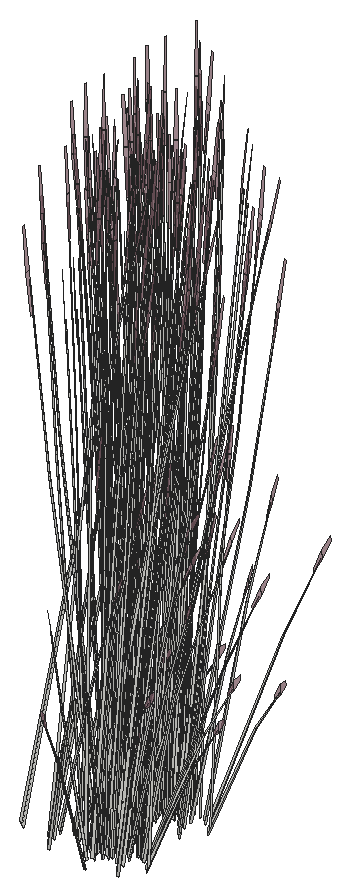
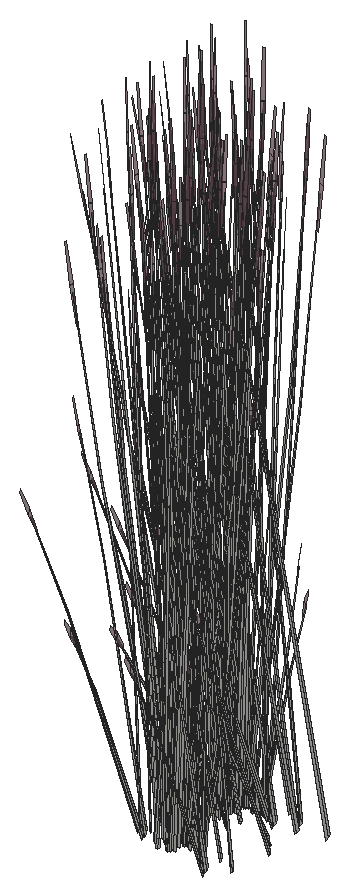
# SketchUp Ruby script. Lengths in inches.
U = 1.inch
M = Sketchup.active_model
def pt(a) = Geom::Point3d.new(a.map { |v| v * U })
def face(e, loops, mat)
  f = e.add_face(loops[0].map { |a| pt(a) })
  loops[1..].each { |l| e.add_face(l.map { |a| pt(a) }).erase! }
  f.material = f.back_material = mat if mat
  f
end
# faces: each face lists its corners as indices into pts; further lists are holes
def faces(e, pts, list, mat = nil) = list.each { |f| face(e, (f[0].is_a?(Array) ? f : [f]).map { |l| l.map { |i| pts[i] } }, mat) }
# xy, xz, yz: faces in a plane at the given z, y or x. An outline is a flat list of corners, or four numbers for a rectangle; further outlines are holes
def ring(l) = l.size == 4 ? [[l[0], l[1]], [l[2], l[1]], [l[2], l[3]], [l[0], l[3]]] : l.each_slice(2).to_a
def flat(e, list, mat, &to3) = list.each { |f| face(e, (f[0].is_a?(Array) ? f : [f]).map { |l| ring(l).map { |u, v| to3.(u, v) } }, mat) }
def xy(e, z, list, mat = nil) = flat(e, list, mat) { |x, y| [x, y, z] }
def xz(e, y, list, mat = nil) = flat(e, list, mat) { |x, z| [x, y, z] }
def yz(e, x, list, mat = nil) = flat(e, list, mat) { |y, z| [x, y, z] }
def lines(e, pts, list) = list.each { |a, b| e.add_line(pt(pts[a]), pt(pts[b])) }
# prism: a flat outline (further loops are holes) pulled along v
def prism(e, loops, v, mat = nil)
  f = face(e, loops, mat); d = Geom::Vector3d.new(v.map { |x| x * U })
  f.pushpull(f.normal.samedirection?(d) ? d.length : -d.length)
end
def box(e, o, s, mat = nil) = prism(e, [[o, [o[0] + s[0], o[1], o[2]], [o[0] + s[0], o[1] + s[1], o[2]], [o[0], o[1] + s[1], o[2]]]], [0, 0, s[2]], mat)
def at(x, y, z, deg = 0) = Geom::Transformation.translation(pt([x, y, z])) * Geom::Transformation.rotation(ORIGIN, Z_AXIS, deg.degrees)
def axes(o, x, y, z) = Geom::Transformation.new([*x, 0, *y, 0, *z, 0, *pt(o).to_a, 1])
def part(name) = M.definitions.add(name)
# library, detail: a bought-in or finely detailed component or shape, given as its bounding box
def library(name, o, s) = part(name).tap { |d| box(d.entities, o, s) }
def detail(e, o, s) = box(e.add_group.entities, o, s)
def put(e, d, t, mat = nil) = e.add_instance(d, t).tap { |i| i.material = mat if mat }
def group(e, t, mat = nil) = e.add_group.tap { |g| g.transformation = t; g.material = mat if mat }.entities
root = M.entities
M.materials.add("LightPink_Translucent").color = [144, 107, 117]
M.materials["LightPink_Translucent"].alpha = 0.75
c1 = part("blade")
p = [[2.15,0.21,22],[0,0.17,0],[0.09,0.45,0],[2.18,0.31,22],[2.29,0.31,22],[0.38,0.45,0],
  [2.48,0.24,33],[2.49,0.24,33],[2.48,0.22,33]]
faces(c1.entities,p,[[0,1,2,3],[4,5,2,3],[6,3,4,7],[8,0,3,6]])
c2 = part("seeds")
p = [[0.3,-0.1,1.38],[-0.01,-0.03,1.59],[-0.01,-0.03,0.03],[0.14,-0.07,-0.07],[0.29,-0.03,3],[0.15,0.01,3.11]]
faces(c2.entities,p,[[0,1,2,3],[1,0,4,5]],"LightPink_Translucent")
c3 = part("blade with seeds")
put(c3.entities,c1,at(0,0,0))
put(c3.entities,c2,axes([2.4,0.25,30.99],[1.5799,-0.05474,1.17369],[-0.12525,1.92788,0.29478],[-0.07173,-0.02425,1.56792]))
put(root,c3,axes([340.58,18.31,49.78],[-0.47255,0.19538,-0.43871],[-0.28245,-0.35034,0],[-0.10763,0.0445,1.3917]))
put(root,c3,axes([337.78,16.37,49.78],[0,-0.39075,-0.43871],[0.56491,0,0],[0,-0.089,1.3917]))
put(root,c3,axes([337.78,22.64,49.78],[0,-0.39075,-0.43871],[0.56491,0,0],[0,-0.089,1.3917]))
put(root,c3,axes([338.02,16.73,50.19],[0,0.39075,0.43871],[-0.56491,0,0],[0,-0.089,1.3917]))
put(root,c3,axes([338.02,23,50.19],[0,0.39075,0.43871],[-0.56491,0,0],[0,-0.089,1.3917]))
put(root,c3,axes([340.61,18.21,49.9375],[-0.31175,-0.39292,-0.04544],[0.52815,-0.21836,0.456],[-0.13015,0.03741,1.44584]))
put(root,c3,axes([335.24,22.97,50.1],[0.31568,-0.39156,0],[0.52815,0.21836,-0.456],[0.12029,0.04973,1.44655]))
put(root,c3,axes([335.77,22.8,49.32],[-0.07557,-0.03078,1.55816],[-0.19412,-0.34391,-0.23804],[0.13095,-0.09333,0.26541]))
put(root,c3,axes([340.46,18.16,49.79],[-0.47106,-0.09668,-0.27372],[0.11861,-0.34048,0.27372],[-0.09497,0.03926,1.22797]))
put(root,c3,axes([333.36,16.0625,49.41],[-0.49699,0.15644,1.13921],[-0.15819,-0.44887,0.44265],[0.30518,0.00747,1.29573]))
put(root,c3,axes([339.25,16.82,50.36],[-0.56863,-0.18645,-0.25709],[0.2738,-0.39352,-0.44182],[-0.01787,-0.09662,1.41118]))
put(root,c3,axes([339.25,23.09,50.36],[-0.56863,-0.18645,-0.25709],[0.2738,-0.39352,-0.44182],[-0.01787,-0.09662,1.41118]))
put(root,c3,axes([338.21,18.43,50.49],[0.45869,-0.0692,0.0575],[0.10545,0.27878,-0.76259],[-0.02908,0.14112,0.68355]))
put(root,c3,axes([340.38,17.17,50.36],[0.05884,0.44587,-0.25709],[-0.6128,0.02696,-0.44182],[-0.10791,0.05939,1.41118]))
put(root,c3,axes([335.65,15.37,50.1],[0.31568,-0.39156,0],[0.52815,0.21836,-0.456],[0.12029,0.04973,1.44655]))
put(root,c3,axes([336.18,15.2,49.32],[-0.07557,-0.03078,1.55816],[-0.19412,-0.34391,-0.23804],[0.13095,-0.09333,0.26541]))
put(root,c3,axes([339,16.42,49.85],[-0.20736,-0.4007,-0.61707],[0.59731,-0.14431,-0.16195],[-0.02292,-0.13569,1.36206]))
put(root,c3,axes([339,22.7,49.85],[-0.20736,-0.4007,-0.61707],[0.59731,-0.14431,-0.16195],[-0.02292,-0.13569,1.36206]))
put(root,c3,axes([334.12,20.87,50.29],[-0.1216,-0.0961,1.26356],[0.15822,-0.31792,-0.27174],[0.24603,0.04307,0.54024]))
put(root,c3,axes([337.08,24.19,50],[-0.31304,-0.24986,-0.05733],[0.34284,-0.22894,-0.25992],[0.09714,-0.01612,0.85731]))
put(root,c3,axes([335.93,15.61,49.78],[0.47255,0.19538,-0.43871],[-0.28245,0.35034,0],[0.10763,0.0445,1.3917]))
put(root,c3,axes([338.02,16.375,49.79],[0.35245,-0.2438,-0.27372],[0.35245,0.2438,0.27372],[0,-0.07853,1.22797]))
put(root,c3,axes([338.02,22.65,49.79],[0.35245,-0.2438,-0.27372],[0.35245,0.2438,0.27372],[0,-0.07853,1.22797]))
put(root,c3,axes([335.91,18.39,49.32],[0.03679,-0.05641,1.55816],[0.46313,-0.16615,-0.23804],[0.14041,0.08599,0.26541]))
put(root,c3,axes([339.61,14.8,49.88],[-0.34892,0.22417,-0.0344],[-0.3197,-0.24551,-0.15595],[-0.02251,-0.06957,0.51438]))
put(root,c3,axes([339.61,21.07,49.88],[-0.34892,0.22417,-0.0344],[-0.3197,-0.24551,-0.15595],[-0.02251,-0.06957,0.51438]))
put(root,c3,axes([339.47,17.01,50.09],[0.63817,0.08233,0.40429],[-0.12987,0.46497,0.15865],[-0.09326,-0.0449,1.40366]))
put(root,c3,axes([339.47,23.28,50.09],[0.63817,0.08233,0.40429],[-0.12987,0.46497,0.15865],[-0.09326,-0.0449,1.40366]))
put(root,c3,axes([335.25,16.35,49.82],[0.52523,0.06406,-0.55095],[-0.11084,0.39517,-0.1446],[0.15674,0.04788,1.21613]))
put(root,c3,axes([339.31,16.93,50.4],[-0.24498,0.3521,0.39531],[-0.50902,-0.16945,-0.19025],[0,-0.08116,1.26923]))
put(root,c3,axes([339.31,23.2,50.4],[-0.24498,0.3521,0.39531],[-0.50902,-0.16945,-0.19025],[0,-0.08116,1.26923]))
put(root,c3,axes([337.48,16.59,50],[-0.31304,-0.24986,-0.05733],[0.34284,-0.22894,-0.25992],[0.09714,-0.01612,0.85731]))
put(root,c3,axes([339.13,17.75,50.1875],[0.54257,-0.10371,0.15589],[0.13397,0.38597,0.31002],[-0.04839,-0.05624,1.41735]))
put(root,c3,axes([339.13,24.03,50.1875],[0.54257,-0.10371,0.15589],[0.13397,0.38597,0.31002],[-0.04839,-0.05624,1.41735]))
put(root,c3,axes([339.83,17.82,49.94],[-0.50902,-0.17543,0],[0.24498,-0.36452,0],[0,0,1.43768]))
put(root,c3,axes([339.83,24.09,49.94],[-0.50902,-0.17543,0],[0.24498,-0.36452,0],[0,0,1.43768]))
put(root,c3,axes([341,18.25,50.1],[0.31568,0.39156,0],[-0.52815,0.21836,-0.456],[-0.12029,0.04973,1.44655]))
put(root,c3,axes([340.74,17.77,50.1875],[0.14586,-0.38834,0.15589],[0.53375,0.1099,0.31002],[-0.0922,0.00189,1.41735]))
put(root,c3,axes([340.74,24.05,50.1875],[0.14586,-0.38834,0.15589],[0.53375,0.1099,0.31002],[-0.0922,0.00189,1.41735]))
put(root,c3,axes([340.5,17.26,50.3125],[0.37303,0.23477,0.12794],[-0.31115,0.26487,-0.36534],[-0.08661,0.03581,1.11991]))
put(root,c3,axes([340.36,16.97,50.03],[-0.46965,-0.33633,-0.05417],[0.46994,-0.33653,0],[-0.0164,-0.01174,1.55135]))
put(root,c3,axes([340.36,23.24,50.03],[-0.46965,-0.33633,-0.05417],[0.46994,-0.33653,0],[-0.0164,-0.01174,1.55135]))
put(root,c3,axes([340.49,17.09,50.4],[0.54829,-0.02412,0.39531],[0.04958,0.40041,-0.19025],[-0.09816,0.04058,1.26923]))
put(root,c3,axes([340.49,23.36,50.4],[0.54829,-0.02412,0.39531],[0.04958,0.40041,-0.19025],[-0.09816,0.04058,1.26923]))
put(root,c3,axes([340.62,18.01,50.06],[0.63212,0.12701,0.27176],[-0.15814,0.45398,-0.32244],[-0.10462,0.05682,1.45692]))
put(root,c3,axes([339.7,14.53,49.32],[-0.08469,0.01408,1.55816],[-0.46834,-0.15847,-0.23804],[0.00786,-0.13218,0.26541]))
put(root,c3,axes([339.7,20.8,49.32],[-0.08469,0.01408,1.55816],[-0.46834,-0.15847,-0.23804],[0.00786,-0.13218,0.26541]))
put(root,c3,axes([340.89,17.98,50.19],[0.47255,-0.19538,0.43871],[0.28245,0.35034,0],[-0.10763,0.0445,1.3917]))
put(root,c3,axes([339.42,16.58,50.09],[0.21952,0.43694,0.40429],[-0.62724,0.15194,0.15865],[0.00767,-0.08029,1.40366]))
put(root,c3,axes([339.42,22.85,50.09],[0.21952,0.43694,0.40429],[-0.62724,0.15194,0.15865],[0.00767,-0.08029,1.40366]))
put(root,c3,axes([339.32,16.53,49.95],[0.24498,-0.3521,-0.39531],[0.50902,0.16945,0.19025],[0,-0.08116,1.26923]))
put(root,c3,axes([339.32,22.8,49.95],[0.24498,-0.3521,-0.39531],[0.50902,0.16945,0.19025],[0,-0.08116,1.26923]))
put(root,c3,axes([339.94,17.66,49.95],[-0.16474,-0.33688,0],[0.47043,-0.11798,0],[0,0,1.36402]))
put(root,c3,axes([339.94,23.93,49.95],[-0.16474,-0.33688,0],[0.47043,-0.11798,0],[0,0,1.36402]))
put(root,c3,axes([339.34,18.375,49.32],[0.08172,-0.02126,1.55816],[0.49154,0.11703,-0.23804],[0.01437,0.1319,0.26541]))
put(root,c3,axes([336.15,23.48,50.29],[-0.18038,-0.01157,1.26356],[-0.18479,-0.31048,-0.27174],[0.22159,-0.08783,0.54024]))
put(root,c3,axes([336.49,24.52,49.75],[-0.3252,0.04689,1.25103],[-0.05176,-0.37326,0.07161],[0.22777,-0.0565,0.71188]))
put(root,c3,axes([340.61,17,49.95],[-0.24498,0.3521,-0.39531],[-0.50902,-0.16945,0.19025],[0,0.08116,1.26923]))
put(root,c3,axes([336.84,24.27,49.32],[-0.02639,-0.05932,1.55816],[0.18302,-0.34702,-0.23804],[0.18462,-0.00499,0.26541]))
put(root,c3,axes([336.55,15.89,50.29],[-0.18038,-0.01157,1.26356],[-0.18479,-0.31048,-0.27174],[0.22159,-0.08783,0.54024]))
put(root,c3,axes([341.58,16.78,50.1875],[-0.39671,-0.28463,0.15589],[0.39978,-0.27607,0.31002],[-0.04381,0.05813,1.41735]))
put(root,c3,axes([341.58,23.06,50.1875],[-0.39671,-0.28463,0.15589],[0.39978,-0.27607,0.31002],[-0.04381,0.05813,1.41735]))
put(root,c3,axes([340.21,16.62,49.95],[0,-0.45213,0],[0.63136,0,0],[0,0,1.58567]))
put(root,c3,axes([340.21,22.89,49.95],[0,-0.45213,0],[0.63136,0,0],[0,0,1.58567]))
put(root,c3,axes([339.62,16.7,50.15],[0.56891,0.18939,0.21263],[-0.2738,0.39352,0.44182],[0,-0.09071,1.41855]))
put(root,c3,axes([339.62,22.97,50.15],[0.56891,0.18939,0.21263],[-0.2738,0.39352,0.44182],[0,-0.09071,1.41855]))
put(root,c3,axes([340.52,16.8,50.03],[0,0.45191,-0.04981],[-0.63136,0,0],[0,0.0142,1.58489]))
put(root,c3,axes([340.52,23.07,50.03],[0,0.45191,-0.04981],[-0.63136,0,0],[0,0.0142,1.58489]))
put(root,c3,axes([339.44,16.4375,50.4],[-0.54829,0.02412,0.39531],[-0.04958,-0.40041,-0.19025],[0.09816,-0.04058,1.26923]))
put(root,c3,axes([339.44,22.71,50.4],[-0.54829,0.02412,0.39531],[-0.04958,-0.40041,-0.19025],[0.09816,-0.04058,1.26923]))
put(root,c3,axes([339.18,15.75,50.1875],[-0.14586,0.38834,0.15589],[-0.53375,-0.1099,0.31002],[0.0922,-0.00189,1.41735]))
put(root,c3,axes([339.18,22.02,50.1875],[-0.14586,0.38834,0.15589],[-0.53375,-0.1099,0.31002],[0.0922,-0.00189,1.41735]))
put(root,c3,axes([336.89,16.92,49.75],[-0.3252,0.04689,1.25103],[-0.05176,-0.37326,0.07161],[0.22777,-0.0565,0.71188]))
put(root,c3,axes([340.22,17.67,50.02],[0.21952,0.44891,-0.05313],[-0.62724,0.1573,0],[0.00767,0.01568,1.52132]))
put(root,c3,axes([337.24,16.67,49.32],[-0.02639,-0.05932,1.55816],[0.18302,-0.34702,-0.23804],[0.18462,-0.00499,0.26541]))
put(root,c3,axes([338.92,15.27,50.1],[-0.31568,-0.39156,0],[0.52815,-0.21836,-0.456],[0.12029,-0.04973,1.44655]))
put(root,c3,axes([338.92,21.54,50.1],[-0.31568,-0.39156,0],[0.52815,-0.21836,-0.456],[0.12029,-0.04973,1.44655]))
put(root,c3,axes([342.03,17.09,49.94],[-0.63105,-0.00312,-0.04397],[0,-0.43672,0.44129],[-0.01983,0.09942,1.3992]))
put(root,c3,axes([340.79,15.77,50.1875],[-0.54257,0.10371,0.15589],[-0.13397,-0.38597,0.31002],[0.04839,0.05624,1.41735]))
put(root,c3,axes([340.79,22.04,50.1875],[-0.54257,0.10371,0.15589],[-0.13397,-0.38597,0.31002],[0.04839,0.05624,1.41735]))
put(root,c3,axes([339.91,16.33,50.09],[-0.41865,0.35461,0.40429],[-0.49737,-0.31303,0.15865],[0.10093,-0.03539,1.40366]))
put(root,c3,axes([339.91,22.61,50.09],[-0.41865,0.35461,0.40429],[-0.49737,-0.31303,0.15865],[0.10093,-0.03539,1.40366]))
put(root,c3,axes([340.62,16.89,49.96],[0.35245,0.2524,0],[-0.35245,0.2524,0],[0,0,1.49564]))
put(root,c3,axes([340.62,23.17,49.96],[0.35245,0.2524,0],[-0.35245,0.2524,0],[0,0,1.49564]))
put(root,c3,axes([340.62,16.6,50.4],[0.24498,-0.3521,0.39531],[0.50902,0.16945,-0.19025],[0,0.08116,1.26923]))
put(root,c3,axes([340.62,22.87,50.4],[0.24498,-0.3521,0.39531],[0.50902,0.16945,-0.19025],[0,0.08116,1.26923]))
put(root,c3,axes([340.4,17.82,49.95],[0.50902,0.17543,0],[-0.24498,0.36452,0],[0,0,1.54589]))
put(root,c3,axes([340.45,16.51,50.1],[-0.63817,-0.08233,0.43472],[0.12987,-0.46497,0.17059],[0.09326,0.0449,1.50931]))
put(root,c3,axes([340.45,22.79,50.1],[-0.63817,-0.08233,0.43472],[0.12987,-0.46497,0.17059],[0.09326,0.0449,1.50931]))
put(root,c3,axes([336.98,17.47,50.29],[-0.1216,-0.0961,1.26356],[0.15822,-0.31792,-0.27174],[0.24603,0.04307,0.54024]))
put(root,c3,axes([341.9,17.15,49.79],[-0.35245,0.2438,-0.27372],[-0.35245,-0.2438,0.27372],[0,0.07853,1.22797]))
put(root,c3,axes([340.9,17.1,49.85],[0.18514,0.35777,-0.61156],[-0.53331,0.12885,-0.16051],[0.02046,0.12115,1.3499]))
put(root,c3,axes([340.63,16.72,49.95],[0.56491,0,0],[0,0.40454,0],[0,0,1.5764]))
put(root,c3,axes([340.63,22.99,49.95],[0.56491,0,0],[0,0.40454,0],[0,0,1.5764]))
put(root,c3,axes([340.09,16.27,50.4],[-0.30332,-0.32798,0.39531],[0.45944,-0.23096,-0.19025],[0.09816,0.04058,1.26923]))
put(root,c3,axes([340.09,22.55,50.4],[-0.30332,-0.32798,0.39531],[0.45944,-0.23096,-0.19025],[0.09816,0.04058,1.26923]))
put(root,c3,axes([339.54,16.35,50.36],[-0.05884,-0.44587,-0.25709],[0.6128,-0.02696,-0.44182],[0.10791,-0.05939,1.41118]))
put(root,c3,axes([339.54,22.625,50.36],[-0.05884,-0.44587,-0.25709],[0.6128,-0.02696,-0.44182],[0.10791,-0.05939,1.41118]))
put(root,c3,axes([340.83,16.68,50.3125],[0.47043,-0.11396,0.12794],[0.16474,0.32541,-0.36534],[0,0.07162,1.11991]))
put(root,c3,axes([340.83,22.95,50.3125],[0.47043,-0.11396,0.12794],[0.16474,0.32541,-0.36534],[0,0.07162,1.11991]))
put(root,c3,axes([340.67,16.71,50.36],[0.56863,0.18645,-0.25709],[-0.2738,0.39352,-0.44182],[0.01787,0.09662,1.41118]))
put(root,c3,axes([339.46,15.37,49.79],[0.47106,0.09668,-0.27372],[-0.11861,0.34048,0.27372],[0.09497,-0.03926,1.22797]))
put(root,c3,axes([339.46,21.64,49.79],[0.47106,0.09668,-0.27372],[-0.11861,0.34048,0.27372],[0.09497,-0.03926,1.22797]))
put(root,c3,axes([340.77,14.96,50.29],[-0.14352,0.07909,1.26356],[-0.42983,-0.13843,-0.27174],[0.07968,-0.17216,0.54024]))
put(root,c3,axes([340.77,21.23,50.29],[-0.14352,0.07909,1.26356],[-0.42983,-0.13843,-0.27174],[0.07968,-0.17216,0.54024]))
put(root,c3,axes([341.9,16.8,50.19],[0,-0.39075,0.43871],[0.56491,0,0],[0,0.089,1.3917]))
put(root,c3,axes([341.9,23.07,50.19],[0,-0.39075,0.43871],[0.56491,0,0],[0,0.089,1.3917]))
put(root,c3,axes([342.15,17.16,49.78],[0,0.39075,-0.43871],[-0.56491,0,0],[0,0.089,1.3917]))
put(root,c3,axes([339.35,15.21,49.78],[0.47255,-0.19538,-0.43871],[0.28245,0.35034,0],[0.10763,-0.0445,1.3917]))
put(root,c3,axes([339.35,21.48,49.78],[0.47255,-0.19538,-0.43871],[0.28245,0.35034,0],[0.10763,-0.0445,1.3917]))
put(root,c3,axes([340.29,16.18,50.3125],[0.09741,-0.34873,0.12794],[0.4759,0.06053,-0.36534],[0.08661,0.03581,1.11991]))
put(root,c3,axes([340.29,22.45,50.3125],[0.09741,-0.34873,0.12794],[0.4759,0.06053,-0.36534],[0.08661,0.03581,1.11991]))
put(root,c3,axes([340.97,15.57,50.19],[-0.47255,-0.19538,0.43871],[0.28245,-0.35034,0],[0.10763,0.0445,1.3917]))
put(root,c3,axes([340.97,21.85,50.19],[-0.47255,-0.19538,0.43871],[0.28245,-0.35034,0],[0.10763,0.0445,1.3917]))
put(root,c3,axes([340.56,17.62,49.93],[0.53009,-0.13258,-0.16963],[0.18627,0.38191,0.00007],[0.05851,-0.01465,1.53656]))
put(root,c3,axes([340.56,23.89,49.93],[0.53009,-0.13258,-0.16963],[0.18627,0.38191,0.00007],[0.05851,-0.01465,1.53656]))
put(root,c3,axes([340.57,16.48,49.95],[0.30332,0.32798,-0.39531],[-0.45944,0.23096,0.19025],[0.09816,0.04058,1.26923]))
put(root,c3,axes([340.57,22.75,49.95],[0.30332,0.32798,-0.39531],[-0.45944,0.23096,0.19025],[0.09816,0.04058,1.26923]))
put(root,c3,axes([340.42,17.85,50.29],[0.00891,-0.12953,1.26356],[0.4258,-0.14469,-0.27174],[0.13144,0.15503,0.54024]))
put(root,c3,axes([339.91,16.01,49.82],[0.34009,-0.2937,-0.55095],[0.42248,0.26632,-0.1446],[0.13628,-0.07327,1.21613]))
put(root,c3,axes([339.91,22.28,49.82],[0.34009,-0.2937,-0.55095],[0.42248,0.26632,-0.1446],[0.13628,-0.07327,1.21613]))
put(root,c3,axes([341.4,15.75,49.79],[0.11861,0.34048,-0.27372],[-0.47106,0.09668,0.27372],[0.09497,0.03926,1.22797]))
put(root,c3,axes([341.4,22.02,49.79],[0.11861,0.34048,-0.27372],[-0.47106,0.09668,0.27372],[0.09497,0.03926,1.22797]))
put(root,c3,axes([342.29,16.86,50.1],[0.63136,0,0],[0,0.43672,-0.456],[0,0.09947,1.44655]))
put(root,c3,axes([340.25,16.3,50.36],[0.50979,-0.25942,-0.25709],[0.339,0.36656,-0.44182],[0.12578,0.03723,1.41118]))
put(root,c3,axes([340.25,22.57,50.36],[0.50979,-0.25942,-0.25709],[0.339,0.36656,-0.44182],[0.12578,0.03723,1.41118]))
put(root,c3,axes([341.47,18.48,50.36],[-0.32378,-0.01225,0.92831],[0.21383,-0.26028,0.51254],[0.12791,0.09247,0.72818]))
put(root,c3,axes([338.96,16.0625,49.41],[-0.49699,0.15644,1.13921],[-0.15819,-0.44887,0.44265],[0.30518,0.00747,1.29573]))
put(root,c3,axes([338.96,22.34,49.41],[-0.49699,0.15644,1.13921],[-0.15819,-0.44887,0.44265],[0.30518,0.00747,1.29573]))
put(root,c3,axes([341.24,15.37,50.1],[0.31568,-0.39156,0],[0.52815,0.21836,-0.456],[0.12029,0.04973,1.44655]))
put(root,c3,axes([341.24,21.64,50.1],[0.31568,-0.39156,0],[0.52815,0.21836,-0.456],[0.12029,0.04973,1.44655]))
put(root,c3,axes([341.77,15.2,49.32],[-0.07557,-0.03078,1.55816],[-0.19412,-0.34391,-0.23804],[0.13095,-0.09333,0.26541]))
put(root,c3,axes([341.77,21.47,49.32],[-0.07557,-0.03078,1.55816],[-0.19412,-0.34391,-0.23804],[0.13095,-0.09333,0.26541]))
put(root,c3,axes([341.53,15.61,49.78],[0.47255,0.19538,-0.43871],[-0.28245,0.35034,0],[0.10763,0.0445,1.3917]))
put(root,c3,axes([341.53,21.88,49.78],[0.47255,0.19538,-0.43871],[-0.28245,0.35034,0],[0.10763,0.0445,1.3917]))
put(root,c3,axes([341.51,18.39,49.32],[0.03679,-0.05641,1.55816],[0.46313,-0.16615,-0.23804],[0.14041,0.08599,0.26541]))
put(root,c3,axes([340.84,16.35,49.82],[0.52523,0.06406,-0.55095],[-0.11084,0.39517,-0.1446],[0.15674,0.04788,1.21613]))
put(root,c3,axes([340.84,22.625,49.82],[0.52523,0.06406,-0.55095],[-0.11084,0.39517,-0.1446],[0.15674,0.04788,1.21613]))
put(root,c3,axes([343.08,16.59,50],[-0.31304,-0.24986,-0.05733],[0.34284,-0.22894,-0.25992],[0.09714,-0.01612,0.85731]))
put(root,c3,axes([343.08,22.86,50],[-0.31304,-0.24986,-0.05733],[0.34284,-0.22894,-0.25992],[0.09714,-0.01612,0.85731]))
put(root,c3,axes([342.15,15.89,50.29],[-0.18038,-0.01157,1.26356],[-0.18479,-0.31048,-0.27174],[0.22159,-0.08783,0.54024]))
put(root,c3,axes([342.15,22.16,50.29],[-0.18038,-0.01157,1.26356],[-0.18479,-0.31048,-0.27174],[0.22159,-0.08783,0.54024]))
put(root,c3,axes([342.49,16.92,49.75],[-0.3252,0.04689,1.25103],[-0.05176,-0.37326,0.07161],[0.22777,-0.0565,0.71188]))
put(root,c3,axes([342.49,23.19,49.75],[-0.3252,0.04689,1.25103],[-0.05176,-0.37326,0.07161],[0.22777,-0.0565,0.71188]))
put(root,c3,axes([342.84,16.67,49.32],[-0.02639,-0.05932,1.55816],[0.18302,-0.34702,-0.23804],[0.18462,-0.00499,0.26541]))
put(root,c3,axes([342.84,22.95,49.32],[-0.02639,-0.05932,1.55816],[0.18302,-0.34702,-0.23804],[0.18462,-0.00499,0.26541]))
put(root,c3,axes([342.58,17.47,50.29],[-0.1216,-0.0961,1.26356],[0.15822,-0.31792,-0.27174],[0.24603,0.04307,0.54024]))
put(root,c3,axes([342.58,23.74,50.29],[-0.1216,-0.0961,1.26356],[0.15822,-0.31792,-0.27174],[0.24603,0.04307,0.54024]))
